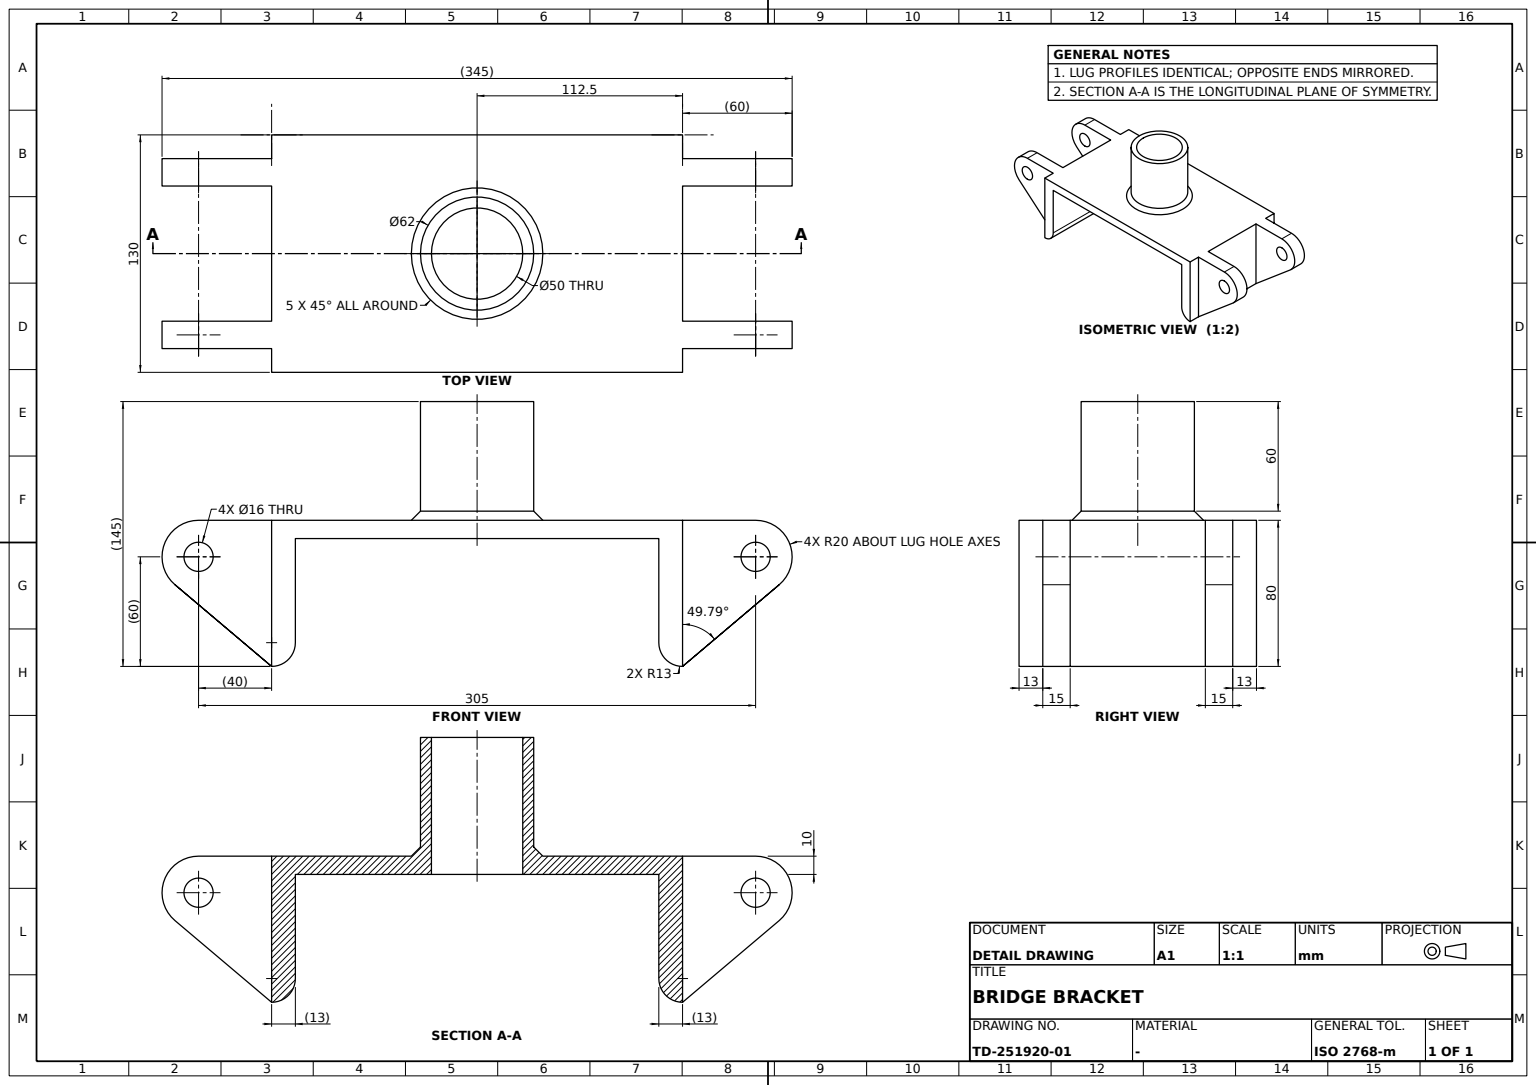
ISO-10303-21;
HEADER;
FILE_DESCRIPTION((''),'2;1');
FILE_NAME('','',(''),(''),'','','');
FILE_SCHEMA(('AUTOMOTIVE_DESIGN'));
ENDSEC;
DATA;
#1=APPLICATION_CONTEXT('');
#2=PRODUCT_CONTEXT('',#1,'mechanical');
#3=PRODUCT('','','',(#2));
#4=PRODUCT_DEFINITION_FORMATION('','',#3);
#5=PRODUCT_DEFINITION_CONTEXT('',#1,'design');
#6=PRODUCT_DEFINITION('','',#4,#5);
#7=PRODUCT_DEFINITION_SHAPE('','',#6);
#8=(LENGTH_UNIT()NAMED_UNIT(*)SI_UNIT(.MILLI.,.METRE.));
#9=(NAMED_UNIT(*)PLANE_ANGLE_UNIT()SI_UNIT($,.RADIAN.));
#10=(NAMED_UNIT(*)SI_UNIT($,.STERADIAN.)SOLID_ANGLE_UNIT());
#11=UNCERTAINTY_MEASURE_WITH_UNIT(LENGTH_MEASURE(0.005),#8,'distance_accuracy_value','');
#12=(GEOMETRIC_REPRESENTATION_CONTEXT(3)GLOBAL_UNCERTAINTY_ASSIGNED_CONTEXT((#11))GLOBAL_UNIT_ASSIGNED_CONTEXT((#8,#9,#10))REPRESENTATION_CONTEXT('',''));
#13=CARTESIAN_POINT('',(-25.,0.,-10.));
#14=VERTEX_POINT('',#13);
#15=CARTESIAN_POINT('',(25.,0.,-10.));
#16=VERTEX_POINT('',#15);
#17=CARTESIAN_POINT('',(0.,0.,-10.));
#18=DIRECTION('',(0.,0.,1.));
#19=DIRECTION('',(1.,0.,0.));
#20=AXIS2_PLACEMENT_3D('',#17,#18,#19);
#21=CIRCLE('',#20,25.);
#22=EDGE_CURVE('',#14,#16,#21,.T.);
#23=ORIENTED_EDGE('',*,*,#22,.F.);
#24=CARTESIAN_POINT('',(-25.,0.,65.));
#25=VERTEX_POINT('',#24);
#26=CARTESIAN_POINT('',(-25.,0.,0.));
#27=VECTOR('',#18,1000.);
#28=LINE('',#26,#27);
#29=EDGE_CURVE('',#14,#25,#28,.T.);
#30=ORIENTED_EDGE('',*,*,#29,.T.);
#31=CARTESIAN_POINT('',(25.,0.,65.));
#32=VERTEX_POINT('',#31);
#33=CARTESIAN_POINT('',(0.,0.,65.));
#34=AXIS2_PLACEMENT_3D('',#33,#18,#19);
#35=CIRCLE('',#34,25.);
#36=EDGE_CURVE('',#25,#32,#35,.T.);
#37=ORIENTED_EDGE('',*,*,#36,.T.);
#38=CARTESIAN_POINT('',(25.,0.,0.));
#39=LINE('',#38,#27);
#40=EDGE_CURVE('',#32,#16,#39,.F.);
#41=ORIENTED_EDGE('',*,*,#40,.T.);
#42=EDGE_LOOP('',(#23,#30,#37,#41));
#43=FACE_BOUND('',#42,.T.);
#44=CARTESIAN_POINT('',(0.,0.,0.));
#45=AXIS2_PLACEMENT_3D('',#44,#18,#19);
#46=CYLINDRICAL_SURFACE('',#45,25.);
#47=ADVANCED_FACE('',(#43),#46,.F.);
#48=CARTESIAN_POINT('',(165.411238,-37.,-35.274159));
#49=VERTEX_POINT('',#48);
#50=CARTESIAN_POINT('',(165.411238,-52.,-35.274159));
#51=VERTEX_POINT('',#50);
#52=DIRECTION('',(0.,-1.,0.));
#53=VECTOR('',#52,1000.);
#54=LINE('',#48,#53);
#55=EDGE_CURVE('',#49,#51,#54,.T.);
#56=ORIENTED_EDGE('',*,*,#55,.F.);
#57=CARTESIAN_POINT('',(152.5,-37.,0.));
#58=VERTEX_POINT('',#57);
#59=CARTESIAN_POINT('',(152.5,-37.,-20.));
#60=AXIS2_PLACEMENT_3D('',#59,#52,#19);
#61=CIRCLE('',#60,20.);
#62=EDGE_CURVE('',#49,#58,#61,.T.);
#63=ORIENTED_EDGE('',*,*,#62,.T.);
#64=CARTESIAN_POINT('',(152.5,-52.,0.));
#65=VERTEX_POINT('',#64);
#66=LINE('',#57,#53);
#67=EDGE_CURVE('',#58,#65,#66,.T.);
#68=ORIENTED_EDGE('',*,*,#67,.T.);
#69=CARTESIAN_POINT('',(152.5,-52.,-20.));
#70=AXIS2_PLACEMENT_3D('',#69,#52,#19);
#71=CIRCLE('',#70,20.);
#72=EDGE_CURVE('',#51,#65,#71,.T.);
#73=ORIENTED_EDGE('',*,*,#72,.F.);
#74=EDGE_LOOP('',(#56,#63,#68,#73));
#75=FACE_BOUND('',#74,.T.);
#76=DIRECTION('',(0.,0.,-1.));
#77=AXIS2_PLACEMENT_3D('',#59,#52,#76);
#78=CYLINDRICAL_SURFACE('',#77,20.);
#79=ADVANCED_FACE('',(#75),#78,.T.);
#80=CARTESIAN_POINT('',(152.5,37.,-12.));
#81=VERTEX_POINT('',#80);
#82=CARTESIAN_POINT('',(152.5,37.,-28.));
#83=VERTEX_POINT('',#82);
#84=CARTESIAN_POINT('',(152.5,37.,-20.));
#85=AXIS2_PLACEMENT_3D('',#84,#52,#19);
#86=CIRCLE('',#85,8.);
#87=EDGE_CURVE('',#81,#83,#86,.T.);
#88=ORIENTED_EDGE('',*,*,#87,.T.);
#89=CARTESIAN_POINT('',(152.5,52.,-28.));
#90=VERTEX_POINT('',#89);
#91=DIRECTION('',(0.,1.,0.));
#92=VECTOR('',#91,1000.);
#93=LINE('',#82,#92);
#94=EDGE_CURVE('',#83,#90,#93,.T.);
#95=ORIENTED_EDGE('',*,*,#94,.T.);
#96=CARTESIAN_POINT('',(152.5,52.,-12.));
#97=VERTEX_POINT('',#96);
#98=CARTESIAN_POINT('',(152.5,52.,-20.));
#99=AXIS2_PLACEMENT_3D('',#98,#52,#19);
#100=CIRCLE('',#99,8.);
#101=EDGE_CURVE('',#97,#90,#100,.T.);
#102=ORIENTED_EDGE('',*,*,#101,.F.);
#103=LINE('',#80,#92);
#104=EDGE_CURVE('',#97,#81,#103,.F.);
#105=ORIENTED_EDGE('',*,*,#104,.T.);
#106=EDGE_LOOP('',(#88,#95,#102,#105));
#107=FACE_BOUND('',#106,.T.);
#108=AXIS2_PLACEMENT_3D('',#84,#91,#18);
#109=CYLINDRICAL_SURFACE('',#108,8.);
#110=ADVANCED_FACE('',(#107),#109,.F.);
#111=EDGE_CURVE('',#32,#25,#35,.T.);
#112=ORIENTED_EDGE('',*,*,#111,.F.);
#113=ORIENTED_EDGE('',*,*,#36,.F.);
#114=EDGE_LOOP('',(#112,#113));
#115=FACE_BOUND('',#114,.T.);
#116=CARTESIAN_POINT('',(-31.,0.,65.));
#117=VERTEX_POINT('',#116);
#118=CARTESIAN_POINT('',(31.,0.,65.));
#119=VERTEX_POINT('',#118);
#120=CIRCLE('',#34,31.);
#121=EDGE_CURVE('',#117,#119,#120,.T.);
#122=ORIENTED_EDGE('',*,*,#121,.T.);
#123=EDGE_CURVE('',#119,#117,#120,.T.);
#124=ORIENTED_EDGE('',*,*,#123,.T.);
#125=EDGE_LOOP('',(#122,#124));
#126=FACE_BOUND('',#125,.T.);
#127=PLANE('',#34);
#128=ADVANCED_FACE('',(#115,#126),#127,.T.);
#129=CARTESIAN_POINT('',(-152.5,-37.,-28.));
#130=VERTEX_POINT('',#129);
#131=CARTESIAN_POINT('',(-152.5,-52.,-28.));
#132=VERTEX_POINT('',#131);
#133=LINE('',#129,#53);
#134=EDGE_CURVE('',#130,#132,#133,.T.);
#135=ORIENTED_EDGE('',*,*,#134,.T.);
#136=CARTESIAN_POINT('',(-152.5,-52.,-12.));
#137=VERTEX_POINT('',#136);
#138=CARTESIAN_POINT('',(-152.5,-52.,-20.));
#139=DIRECTION('',(-1.,0.,0.));
#140=AXIS2_PLACEMENT_3D('',#138,#91,#139);
#141=CIRCLE('',#140,8.);
#142=EDGE_CURVE('',#137,#132,#141,.T.);
#143=ORIENTED_EDGE('',*,*,#142,.F.);
#144=CARTESIAN_POINT('',(-152.5,-37.,-12.));
#145=VERTEX_POINT('',#144);
#146=LINE('',#144,#53);
#147=EDGE_CURVE('',#137,#145,#146,.F.);
#148=ORIENTED_EDGE('',*,*,#147,.T.);
#149=CARTESIAN_POINT('',(-152.5,-37.,-20.));
#150=AXIS2_PLACEMENT_3D('',#149,#91,#139);
#151=CIRCLE('',#150,8.);
#152=EDGE_CURVE('',#145,#130,#151,.T.);
#153=ORIENTED_EDGE('',*,*,#152,.T.);
#154=EDGE_LOOP('',(#135,#143,#148,#153));
#155=FACE_BOUND('',#154,.T.);
#156=AXIS2_PLACEMENT_3D('',#149,#52,#76);
#157=CYLINDRICAL_SURFACE('',#156,8.);
#158=ADVANCED_FACE('',(#155),#157,.F.);
#159=CARTESIAN_POINT('',(-152.5,37.,-12.));
#160=VERTEX_POINT('',#159);
#161=CARTESIAN_POINT('',(-152.5,37.,-28.));
#162=VERTEX_POINT('',#161);
#163=CARTESIAN_POINT('',(-152.5,37.,-20.));
#164=AXIS2_PLACEMENT_3D('',#163,#91,#139);
#165=CIRCLE('',#164,8.);
#166=EDGE_CURVE('',#160,#162,#165,.T.);
#167=ORIENTED_EDGE('',*,*,#166,.F.);
#168=CARTESIAN_POINT('',(-152.5,52.,-12.));
#169=VERTEX_POINT('',#168);
#170=LINE('',#159,#92);
#171=EDGE_CURVE('',#160,#169,#170,.T.);
#172=ORIENTED_EDGE('',*,*,#171,.T.);
#173=CARTESIAN_POINT('',(-152.5,52.,-28.));
#174=VERTEX_POINT('',#173);
#175=CARTESIAN_POINT('',(-152.5,52.,-20.));
#176=AXIS2_PLACEMENT_3D('',#175,#91,#139);
#177=CIRCLE('',#176,8.);
#178=EDGE_CURVE('',#169,#174,#177,.T.);
#179=ORIENTED_EDGE('',*,*,#178,.T.);
#180=LINE('',#161,#92);
#181=EDGE_CURVE('',#174,#162,#180,.F.);
#182=ORIENTED_EDGE('',*,*,#181,.T.);
#183=EDGE_LOOP('',(#167,#172,#179,#182));
#184=FACE_BOUND('',#183,.T.);
#185=AXIS2_PLACEMENT_3D('',#163,#91,#18);
#186=CYLINDRICAL_SURFACE('',#185,8.);
#187=ADVANCED_FACE('',(#184),#186,.F.);
#188=CARTESIAN_POINT('',(112.5,65.,-80.));
#189=VERTEX_POINT('',#188);
#190=CARTESIAN_POINT('',(112.5,65.,0.));
#191=VERTEX_POINT('',#190);
#192=LINE('',#188,#27);
#193=EDGE_CURVE('',#189,#191,#192,.T.);
#194=ORIENTED_EDGE('',*,*,#193,.F.);
#195=CARTESIAN_POINT('',(99.5,65.,-67.));
#196=VERTEX_POINT('',#195);
#197=CARTESIAN_POINT('',(112.5,65.,-67.));
#198=AXIS2_PLACEMENT_3D('',#197,#52,#19);
#199=CIRCLE('',#198,13.);
#200=EDGE_CURVE('',#196,#189,#199,.T.);
#201=ORIENTED_EDGE('',*,*,#200,.F.);
#202=CARTESIAN_POINT('',(99.5,65.,-10.));
#203=VERTEX_POINT('',#202);
#204=VECTOR('',#76,1000.);
#205=LINE('',#202,#204);
#206=EDGE_CURVE('',#203,#196,#205,.T.);
#207=ORIENTED_EDGE('',*,*,#206,.F.);
#208=CARTESIAN_POINT('',(-99.5,65.,-10.));
#209=VERTEX_POINT('',#208);
#210=VECTOR('',#19,1000.);
#211=LINE('',#208,#210);
#212=EDGE_CURVE('',#209,#203,#211,.T.);
#213=ORIENTED_EDGE('',*,*,#212,.F.);
#214=CARTESIAN_POINT('',(-99.5,65.,-67.));
#215=VERTEX_POINT('',#214);
#216=LINE('',#214,#27);
#217=EDGE_CURVE('',#215,#209,#216,.T.);
#218=ORIENTED_EDGE('',*,*,#217,.F.);
#219=CARTESIAN_POINT('',(-112.5,65.,-80.));
#220=VERTEX_POINT('',#219);
#221=CARTESIAN_POINT('',(-112.5,65.,-67.));
#222=AXIS2_PLACEMENT_3D('',#221,#52,#19);
#223=CIRCLE('',#222,13.);
#224=EDGE_CURVE('',#220,#215,#223,.T.);
#225=ORIENTED_EDGE('',*,*,#224,.F.);
#226=CARTESIAN_POINT('',(-112.5,65.,0.));
#227=VERTEX_POINT('',#226);
#228=LINE('',#226,#204);
#229=EDGE_CURVE('',#227,#220,#228,.T.);
#230=ORIENTED_EDGE('',*,*,#229,.F.);
#231=VECTOR('',#139,1000.);
#232=LINE('',#190,#231);
#233=EDGE_CURVE('',#191,#227,#232,.T.);
#234=ORIENTED_EDGE('',*,*,#233,.F.);
#235=EDGE_LOOP('',(#194,#201,#207,#213,#218,#225,#230,#234));
#236=FACE_BOUND('',#235,.T.);
#237=AXIS2_PLACEMENT_3D('',#221,#52,#76);
#238=PLANE('',#237);
#239=ADVANCED_FACE('',(#236),#238,.F.);
#240=ORIENTED_EDGE('',*,*,#181,.F.);
#241=EDGE_CURVE('',#174,#169,#177,.T.);
#242=ORIENTED_EDGE('',*,*,#241,.T.);
#243=ORIENTED_EDGE('',*,*,#171,.F.);
#244=EDGE_CURVE('',#162,#160,#165,.T.);
#245=ORIENTED_EDGE('',*,*,#244,.F.);
#246=EDGE_LOOP('',(#240,#242,#243,#245));
#247=FACE_BOUND('',#246,.T.);
#248=ADVANCED_FACE('',(#247),#186,.F.);
#249=CARTESIAN_POINT('',(112.5,-52.,-80.));
#250=VERTEX_POINT('',#249);
#251=DIRECTION('',(0.763707941,0.,0.645561911));
#252=VECTOR('',#251,1000.);
#253=LINE('',#249,#252);
#254=EDGE_CURVE('',#250,#51,#253,.T.);
#255=ORIENTED_EDGE('',*,*,#254,.F.);
#256=CARTESIAN_POINT('',(112.5,-37.,-80.));
#257=VERTEX_POINT('',#256);
#258=LINE('',#256,#53);
#259=EDGE_CURVE('',#257,#250,#258,.T.);
#260=ORIENTED_EDGE('',*,*,#259,.F.);
#261=LINE('',#256,#252);
#262=EDGE_CURVE('',#257,#49,#261,.T.);
#263=ORIENTED_EDGE('',*,*,#262,.T.);
#264=ORIENTED_EDGE('',*,*,#55,.T.);
#265=EDGE_LOOP('',(#255,#260,#263,#264));
#266=FACE_BOUND('',#265,.T.);
#267=DIRECTION('',(0.645561911,0.,-0.763707941));
#268=DIRECTION('',(-0.763707941,0.,-0.645561911));
#269=AXIS2_PLACEMENT_3D('',#256,#267,#268);
#270=PLANE('',#269);
#271=ADVANCED_FACE('',(#266),#270,.T.);
#272=CARTESIAN_POINT('',(152.5,-52.,-12.));
#273=VERTEX_POINT('',#272);
#274=CARTESIAN_POINT('',(152.5,-37.,-12.));
#275=VERTEX_POINT('',#274);
#276=LINE('',#274,#53);
#277=EDGE_CURVE('',#273,#275,#276,.F.);
#278=ORIENTED_EDGE('',*,*,#277,.F.);
#279=CARTESIAN_POINT('',(152.5,-52.,-28.));
#280=VERTEX_POINT('',#279);
#281=CIRCLE('',#70,8.);
#282=EDGE_CURVE('',#273,#280,#281,.T.);
#283=ORIENTED_EDGE('',*,*,#282,.T.);
#284=CARTESIAN_POINT('',(152.5,-37.,-28.));
#285=VERTEX_POINT('',#284);
#286=LINE('',#284,#53);
#287=EDGE_CURVE('',#285,#280,#286,.T.);
#288=ORIENTED_EDGE('',*,*,#287,.F.);
#289=CIRCLE('',#60,8.);
#290=EDGE_CURVE('',#275,#285,#289,.T.);
#291=ORIENTED_EDGE('',*,*,#290,.F.);
#292=EDGE_LOOP('',(#278,#283,#288,#291));
#293=FACE_BOUND('',#292,.T.);
#294=CYLINDRICAL_SURFACE('',#77,8.);
#295=ADVANCED_FACE('',(#293),#294,.F.);
#296=ORIENTED_EDGE('',*,*,#287,.T.);
#297=EDGE_CURVE('',#280,#273,#281,.T.);
#298=ORIENTED_EDGE('',*,*,#297,.T.);
#299=ORIENTED_EDGE('',*,*,#277,.T.);
#300=EDGE_CURVE('',#285,#275,#289,.T.);
#301=ORIENTED_EDGE('',*,*,#300,.F.);
#302=EDGE_LOOP('',(#296,#298,#299,#301));
#303=FACE_BOUND('',#302,.T.);
#304=ADVANCED_FACE('',(#303),#294,.F.);
#305=CARTESIAN_POINT('',(152.5,37.,0.));
#306=VERTEX_POINT('',#305);
#307=CARTESIAN_POINT('',(112.5,37.,0.));
#308=VERTEX_POINT('',#307);
#309=LINE('',#305,#231);
#310=EDGE_CURVE('',#306,#308,#309,.T.);
#311=ORIENTED_EDGE('',*,*,#310,.F.);
#312=CARTESIAN_POINT('',(152.5,52.,0.));
#313=VERTEX_POINT('',#312);
#314=LINE('',#305,#92);
#315=EDGE_CURVE('',#306,#313,#314,.T.);
#316=ORIENTED_EDGE('',*,*,#315,.T.);
#317=CARTESIAN_POINT('',(112.5,52.,0.));
#318=VERTEX_POINT('',#317);
#319=LINE('',#312,#231);
#320=EDGE_CURVE('',#313,#318,#319,.T.);
#321=ORIENTED_EDGE('',*,*,#320,.T.);
#322=CARTESIAN_POINT('',(112.5,-65.,0.));
#323=LINE('',#322,#92);
#324=EDGE_CURVE('',#318,#191,#323,.T.);
#325=ORIENTED_EDGE('',*,*,#324,.T.);
#326=ORIENTED_EDGE('',*,*,#233,.T.);
#327=CARTESIAN_POINT('',(-112.5,52.,0.));
#328=VERTEX_POINT('',#327);
#329=CARTESIAN_POINT('',(-112.5,-65.,0.));
#330=LINE('',#329,#92);
#331=EDGE_CURVE('',#328,#227,#330,.T.);
#332=ORIENTED_EDGE('',*,*,#331,.F.);
#333=CARTESIAN_POINT('',(-152.5,52.,0.));
#334=VERTEX_POINT('',#333);
#335=LINE('',#333,#210);
#336=EDGE_CURVE('',#334,#328,#335,.T.);
#337=ORIENTED_EDGE('',*,*,#336,.F.);
#338=CARTESIAN_POINT('',(-152.5,37.,0.));
#339=VERTEX_POINT('',#338);
#340=LINE('',#338,#92);
#341=EDGE_CURVE('',#339,#334,#340,.T.);
#342=ORIENTED_EDGE('',*,*,#341,.F.);
#343=CARTESIAN_POINT('',(-112.5,37.,0.));
#344=VERTEX_POINT('',#343);
#345=LINE('',#338,#210);
#346=EDGE_CURVE('',#339,#344,#345,.T.);
#347=ORIENTED_EDGE('',*,*,#346,.T.);
#348=CARTESIAN_POINT('',(-112.5,-37.,0.));
#349=VERTEX_POINT('',#348);
#350=EDGE_CURVE('',#349,#344,#330,.T.);
#351=ORIENTED_EDGE('',*,*,#350,.F.);
#352=CARTESIAN_POINT('',(-152.5,-37.,0.));
#353=VERTEX_POINT('',#352);
#354=LINE('',#352,#210);
#355=EDGE_CURVE('',#353,#349,#354,.T.);
#356=ORIENTED_EDGE('',*,*,#355,.F.);
#357=CARTESIAN_POINT('',(-152.5,-52.,0.));
#358=VERTEX_POINT('',#357);
#359=LINE('',#352,#53);
#360=EDGE_CURVE('',#353,#358,#359,.T.);
#361=ORIENTED_EDGE('',*,*,#360,.T.);
#362=CARTESIAN_POINT('',(-112.5,-52.,0.));
#363=VERTEX_POINT('',#362);
#364=LINE('',#357,#210);
#365=EDGE_CURVE('',#358,#363,#364,.T.);
#366=ORIENTED_EDGE('',*,*,#365,.T.);
#367=VERTEX_POINT('',#329);
#368=EDGE_CURVE('',#367,#363,#330,.T.);
#369=ORIENTED_EDGE('',*,*,#368,.F.);
#370=VERTEX_POINT('',#322);
#371=LINE('',#322,#231);
#372=EDGE_CURVE('',#370,#367,#371,.T.);
#373=ORIENTED_EDGE('',*,*,#372,.F.);
#374=CARTESIAN_POINT('',(112.5,-52.,0.));
#375=VERTEX_POINT('',#374);
#376=EDGE_CURVE('',#370,#375,#323,.T.);
#377=ORIENTED_EDGE('',*,*,#376,.T.);
#378=LINE('',#64,#231);
#379=EDGE_CURVE('',#65,#375,#378,.T.);
#380=ORIENTED_EDGE('',*,*,#379,.F.);
#381=ORIENTED_EDGE('',*,*,#67,.F.);
#382=CARTESIAN_POINT('',(112.5,-37.,0.));
#383=VERTEX_POINT('',#382);
#384=LINE('',#57,#231);
#385=EDGE_CURVE('',#58,#383,#384,.T.);
#386=ORIENTED_EDGE('',*,*,#385,.T.);
#387=EDGE_CURVE('',#383,#308,#323,.T.);
#388=ORIENTED_EDGE('',*,*,#387,.T.);
#389=EDGE_LOOP('',(#311,#316,#321,#325,#326,#332,#337,#342,#347,#351,#356,#361,#366,#369,#373,#377,#380,#381,#386,#388));
#390=FACE_BOUND('',#389,.T.);
#391=CARTESIAN_POINT('',(36.,0.,0.));
#392=VERTEX_POINT('',#391);
#393=CARTESIAN_POINT('',(-36.,0.,0.));
#394=VERTEX_POINT('',#393);
#395=AXIS2_PLACEMENT_3D('',#44,#76,#139);
#396=CIRCLE('',#395,36.);
#397=EDGE_CURVE('',#392,#394,#396,.T.);
#398=ORIENTED_EDGE('',*,*,#397,.T.);
#399=EDGE_CURVE('',#394,#392,#396,.T.);
#400=ORIENTED_EDGE('',*,*,#399,.T.);
#401=EDGE_LOOP('',(#398,#400));
#402=FACE_BOUND('',#401,.T.);
#403=AXIS2_PLACEMENT_3D('',#322,#76,#139);
#404=PLANE('',#403);
#405=ADVANCED_FACE('',(#390,#402),#404,.F.);
#406=ORIENTED_EDGE('',*,*,#399,.F.);
#407=CARTESIAN_POINT('',(-31.,0.,5.));
#408=VERTEX_POINT('',#407);
#409=DIRECTION('',(-0.707106781,0.,-0.707106781));
#410=VECTOR('',#409,1000.);
#411=LINE('',#407,#410);
#412=EDGE_CURVE('',#408,#394,#411,.T.);
#413=ORIENTED_EDGE('',*,*,#412,.F.);
#414=CARTESIAN_POINT('',(31.,0.,5.));
#415=VERTEX_POINT('',#414);
#416=CARTESIAN_POINT('',(0.,0.,5.));
#417=AXIS2_PLACEMENT_3D('',#416,#18,#139);
#418=CIRCLE('',#417,31.);
#419=EDGE_CURVE('',#415,#408,#418,.T.);
#420=ORIENTED_EDGE('',*,*,#419,.F.);
#421=DIRECTION('',(0.707106781,0.,-0.707106781));
#422=VECTOR('',#421,1000.);
#423=LINE('',#414,#422);
#424=EDGE_CURVE('',#392,#415,#423,.F.);
#425=ORIENTED_EDGE('',*,*,#424,.F.);
#426=EDGE_LOOP('',(#406,#413,#420,#425));
#427=FACE_BOUND('',#426,.T.);
#428=AXIS2_PLACEMENT_3D('',#416,#76,#139);
#429=CONICAL_SURFACE('',#428,31.,0.785398163);
#430=ADVANCED_FACE('',(#427),#429,.T.);
#431=CARTESIAN_POINT('',(99.5,-65.,-10.));
#432=VERTEX_POINT('',#431);
#433=LINE('',#431,#92);
#434=EDGE_CURVE('',#432,#203,#433,.T.);
#435=ORIENTED_EDGE('',*,*,#434,.F.);
#436=CARTESIAN_POINT('',(-99.5,-65.,-10.));
#437=VERTEX_POINT('',#436);
#438=LINE('',#436,#210);
#439=EDGE_CURVE('',#437,#432,#438,.T.);
#440=ORIENTED_EDGE('',*,*,#439,.F.);
#441=LINE('',#436,#92);
#442=EDGE_CURVE('',#437,#209,#441,.T.);
#443=ORIENTED_EDGE('',*,*,#442,.T.);
#444=ORIENTED_EDGE('',*,*,#212,.T.);
#445=EDGE_LOOP('',(#435,#440,#443,#444));
#446=FACE_BOUND('',#445,.T.);
#447=EDGE_CURVE('',#16,#14,#21,.T.);
#448=ORIENTED_EDGE('',*,*,#447,.T.);
#449=ORIENTED_EDGE('',*,*,#22,.T.);
#450=EDGE_LOOP('',(#448,#449));
#451=FACE_BOUND('',#450,.T.);
#452=AXIS2_PLACEMENT_3D('',#436,#18,#19);
#453=PLANE('',#452);
#454=ADVANCED_FACE('',(#446,#451),#453,.F.);
#455=CARTESIAN_POINT('',(112.5,37.,-80.));
#456=VERTEX_POINT('',#455);
#457=CARTESIAN_POINT('',(112.5,-65.,-80.));
#458=LINE('',#457,#92);
#459=EDGE_CURVE('',#257,#456,#458,.T.);
#460=ORIENTED_EDGE('',*,*,#459,.T.);
#461=LINE('',#307,#204);
#462=EDGE_CURVE('',#308,#456,#461,.T.);
#463=ORIENTED_EDGE('',*,*,#462,.F.);
#464=ORIENTED_EDGE('',*,*,#387,.F.);
#465=LINE('',#382,#204);
#466=EDGE_CURVE('',#383,#257,#465,.T.);
#467=ORIENTED_EDGE('',*,*,#466,.T.);
#468=EDGE_LOOP('',(#460,#463,#464,#467));
#469=FACE_BOUND('',#468,.T.);
#470=AXIS2_PLACEMENT_3D('',#457,#139,#18);
#471=PLANE('',#470);
#472=ADVANCED_FACE('',(#469),#471,.F.);
#473=ORIENTED_EDGE('',*,*,#62,.F.);
#474=ORIENTED_EDGE('',*,*,#262,.F.);
#475=ORIENTED_EDGE('',*,*,#466,.F.);
#476=ORIENTED_EDGE('',*,*,#385,.F.);
#477=EDGE_LOOP('',(#473,#474,#475,#476));
#478=FACE_BOUND('',#477,.T.);
#479=ORIENTED_EDGE('',*,*,#290,.T.);
#480=ORIENTED_EDGE('',*,*,#300,.T.);
#481=EDGE_LOOP('',(#479,#480));
#482=FACE_BOUND('',#481,.T.);
#483=PLANE('',#77);
#484=ADVANCED_FACE('',(#478,#482),#483,.F.);
#485=CARTESIAN_POINT('',(165.411238,52.,-35.274159));
#486=VERTEX_POINT('',#485);
#487=CIRCLE('',#99,20.);
#488=EDGE_CURVE('',#486,#313,#487,.T.);
#489=ORIENTED_EDGE('',*,*,#488,.F.);
#490=CARTESIAN_POINT('',(112.5,52.,-80.));
#491=VERTEX_POINT('',#490);
#492=LINE('',#490,#252);
#493=EDGE_CURVE('',#491,#486,#492,.T.);
#494=ORIENTED_EDGE('',*,*,#493,.F.);
#495=LINE('',#317,#204);
#496=EDGE_CURVE('',#318,#491,#495,.T.);
#497=ORIENTED_EDGE('',*,*,#496,.F.);
#498=ORIENTED_EDGE('',*,*,#320,.F.);
#499=EDGE_LOOP('',(#489,#494,#497,#498));
#500=FACE_BOUND('',#499,.T.);
#501=EDGE_CURVE('',#90,#97,#100,.T.);
#502=ORIENTED_EDGE('',*,*,#501,.T.);
#503=ORIENTED_EDGE('',*,*,#101,.T.);
#504=EDGE_LOOP('',(#502,#503));
#505=FACE_BOUND('',#504,.T.);
#506=AXIS2_PLACEMENT_3D('',#98,#52,#76);
#507=PLANE('',#506);
#508=ADVANCED_FACE('',(#500,#505),#507,.F.);
#509=ORIENTED_EDGE('',*,*,#147,.F.);
#510=EDGE_CURVE('',#132,#137,#141,.T.);
#511=ORIENTED_EDGE('',*,*,#510,.F.);
#512=ORIENTED_EDGE('',*,*,#134,.F.);
#513=EDGE_CURVE('',#130,#145,#151,.T.);
#514=ORIENTED_EDGE('',*,*,#513,.T.);
#515=EDGE_LOOP('',(#509,#511,#512,#514));
#516=FACE_BOUND('',#515,.T.);
#517=ADVANCED_FACE('',(#516),#157,.F.);
#518=ORIENTED_EDGE('',*,*,#341,.T.);
#519=CARTESIAN_POINT('',(-165.411238,52.,-35.274159));
#520=VERTEX_POINT('',#519);
#521=CIRCLE('',#176,20.);
#522=EDGE_CURVE('',#520,#334,#521,.T.);
#523=ORIENTED_EDGE('',*,*,#522,.F.);
#524=CARTESIAN_POINT('',(-165.411238,37.,-35.274159));
#525=VERTEX_POINT('',#524);
#526=LINE('',#524,#92);
#527=EDGE_CURVE('',#525,#520,#526,.T.);
#528=ORIENTED_EDGE('',*,*,#527,.F.);
#529=CIRCLE('',#164,20.);
#530=EDGE_CURVE('',#525,#339,#529,.T.);
#531=ORIENTED_EDGE('',*,*,#530,.T.);
#532=EDGE_LOOP('',(#518,#523,#528,#531));
#533=FACE_BOUND('',#532,.T.);
#534=CYLINDRICAL_SURFACE('',#185,20.);
#535=ADVANCED_FACE('',(#533),#534,.T.);
#536=CARTESIAN_POINT('',(-112.5,-37.,-80.));
#537=VERTEX_POINT('',#536);
#538=LINE('',#348,#204);
#539=EDGE_CURVE('',#349,#537,#538,.T.);
#540=ORIENTED_EDGE('',*,*,#539,.F.);
#541=ORIENTED_EDGE('',*,*,#350,.T.);
#542=CARTESIAN_POINT('',(-112.5,37.,-80.));
#543=VERTEX_POINT('',#542);
#544=LINE('',#343,#204);
#545=EDGE_CURVE('',#344,#543,#544,.T.);
#546=ORIENTED_EDGE('',*,*,#545,.T.);
#547=CARTESIAN_POINT('',(-112.5,-65.,-80.));
#548=LINE('',#547,#92);
#549=EDGE_CURVE('',#537,#543,#548,.T.);
#550=ORIENTED_EDGE('',*,*,#549,.F.);
#551=EDGE_LOOP('',(#540,#541,#546,#550));
#552=FACE_BOUND('',#551,.T.);
#553=AXIS2_PLACEMENT_3D('',#329,#19,#76);
#554=PLANE('',#553);
#555=ADVANCED_FACE('',(#552),#554,.F.);
#556=ORIENTED_EDGE('',*,*,#200,.T.);
#557=EDGE_CURVE('',#491,#189,#458,.T.);
#558=ORIENTED_EDGE('',*,*,#557,.F.);
#559=LINE('',#455,#92);
#560=EDGE_CURVE('',#456,#491,#559,.T.);
#561=ORIENTED_EDGE('',*,*,#560,.F.);
#562=ORIENTED_EDGE('',*,*,#459,.F.);
#563=ORIENTED_EDGE('',*,*,#259,.T.);
#564=VERTEX_POINT('',#457);
#565=EDGE_CURVE('',#564,#250,#458,.T.);
#566=ORIENTED_EDGE('',*,*,#565,.F.);
#567=CARTESIAN_POINT('',(99.5,-65.,-67.));
#568=VERTEX_POINT('',#567);
#569=CARTESIAN_POINT('',(112.5,-65.,-67.));
#570=AXIS2_PLACEMENT_3D('',#569,#52,#19);
#571=CIRCLE('',#570,13.);
#572=EDGE_CURVE('',#568,#564,#571,.T.);
#573=ORIENTED_EDGE('',*,*,#572,.F.);
#574=LINE('',#567,#92);
#575=EDGE_CURVE('',#568,#196,#574,.T.);
#576=ORIENTED_EDGE('',*,*,#575,.T.);
#577=EDGE_LOOP('',(#556,#558,#561,#562,#563,#566,#573,#576));
#578=FACE_BOUND('',#577,.T.);
#579=AXIS2_PLACEMENT_3D('',#569,#91,#18);
#580=CYLINDRICAL_SURFACE('',#579,13.);
#581=ADVANCED_FACE('',(#578),#580,.T.);
#582=VERTEX_POINT('',#547);
#583=LINE('',#329,#204);
#584=EDGE_CURVE('',#367,#582,#583,.T.);
#585=ORIENTED_EDGE('',*,*,#584,.F.);
#586=ORIENTED_EDGE('',*,*,#368,.T.);
#587=CARTESIAN_POINT('',(-112.5,-52.,-80.));
#588=VERTEX_POINT('',#587);
#589=LINE('',#362,#204);
#590=EDGE_CURVE('',#363,#588,#589,.T.);
#591=ORIENTED_EDGE('',*,*,#590,.T.);
#592=EDGE_CURVE('',#582,#588,#548,.T.);
#593=ORIENTED_EDGE('',*,*,#592,.F.);
#594=EDGE_LOOP('',(#585,#586,#591,#593));
#595=FACE_BOUND('',#594,.T.);
#596=ADVANCED_FACE('',(#595),#554,.F.);
#597=LINE('',#374,#204);
#598=EDGE_CURVE('',#375,#250,#597,.T.);
#599=ORIENTED_EDGE('',*,*,#598,.F.);
#600=ORIENTED_EDGE('',*,*,#376,.F.);
#601=LINE('',#457,#27);
#602=EDGE_CURVE('',#564,#370,#601,.T.);
#603=ORIENTED_EDGE('',*,*,#602,.F.);
#604=ORIENTED_EDGE('',*,*,#565,.T.);
#605=EDGE_LOOP('',(#599,#600,#603,#604));
#606=FACE_BOUND('',#605,.T.);
#607=ADVANCED_FACE('',(#606),#471,.F.);
#608=ORIENTED_EDGE('',*,*,#87,.F.);
#609=EDGE_CURVE('',#83,#81,#86,.T.);
#610=ORIENTED_EDGE('',*,*,#609,.F.);
#611=EDGE_LOOP('',(#608,#610));
#612=FACE_BOUND('',#611,.T.);
#613=ORIENTED_EDGE('',*,*,#462,.T.);
#614=CARTESIAN_POINT('',(165.411238,37.,-35.274159));
#615=VERTEX_POINT('',#614);
#616=LINE('',#455,#252);
#617=EDGE_CURVE('',#456,#615,#616,.T.);
#618=ORIENTED_EDGE('',*,*,#617,.T.);
#619=CIRCLE('',#85,20.);
#620=EDGE_CURVE('',#615,#306,#619,.T.);
#621=ORIENTED_EDGE('',*,*,#620,.T.);
#622=ORIENTED_EDGE('',*,*,#310,.T.);
#623=EDGE_LOOP('',(#613,#618,#621,#622));
#624=FACE_BOUND('',#623,.T.);
#625=AXIS2_PLACEMENT_3D('',#84,#52,#76);
#626=PLANE('',#625);
#627=ADVANCED_FACE('',(#612,#624),#626,.T.);
#628=ORIENTED_EDGE('',*,*,#72,.T.);
#629=ORIENTED_EDGE('',*,*,#379,.T.);
#630=ORIENTED_EDGE('',*,*,#598,.T.);
#631=ORIENTED_EDGE('',*,*,#254,.T.);
#632=EDGE_LOOP('',(#628,#629,#630,#631));
#633=FACE_BOUND('',#632,.T.);
#634=ORIENTED_EDGE('',*,*,#297,.F.);
#635=ORIENTED_EDGE('',*,*,#282,.F.);
#636=EDGE_LOOP('',(#634,#635));
#637=FACE_BOUND('',#636,.T.);
#638=AXIS2_PLACEMENT_3D('',#69,#52,#76);
#639=PLANE('',#638);
#640=ADVANCED_FACE('',(#633,#637),#639,.T.);
#641=ORIENTED_EDGE('',*,*,#442,.F.);
#642=CARTESIAN_POINT('',(-99.5,-65.,-67.));
#643=VERTEX_POINT('',#642);
#644=LINE('',#642,#27);
#645=EDGE_CURVE('',#643,#437,#644,.T.);
#646=ORIENTED_EDGE('',*,*,#645,.F.);
#647=LINE('',#642,#92);
#648=EDGE_CURVE('',#643,#215,#647,.T.);
#649=ORIENTED_EDGE('',*,*,#648,.T.);
#650=ORIENTED_EDGE('',*,*,#217,.T.);
#651=EDGE_LOOP('',(#641,#646,#649,#650));
#652=FACE_BOUND('',#651,.T.);
#653=AXIS2_PLACEMENT_3D('',#642,#139,#18);
#654=PLANE('',#653);
#655=ADVANCED_FACE('',(#652),#654,.F.);
#656=ORIENTED_EDGE('',*,*,#360,.F.);
#657=CARTESIAN_POINT('',(-165.411238,-37.,-35.274159));
#658=VERTEX_POINT('',#657);
#659=CIRCLE('',#150,20.);
#660=EDGE_CURVE('',#658,#353,#659,.T.);
#661=ORIENTED_EDGE('',*,*,#660,.F.);
#662=CARTESIAN_POINT('',(-165.411238,-52.,-35.274159));
#663=VERTEX_POINT('',#662);
#664=LINE('',#657,#53);
#665=EDGE_CURVE('',#658,#663,#664,.T.);
#666=ORIENTED_EDGE('',*,*,#665,.T.);
#667=CIRCLE('',#140,20.);
#668=EDGE_CURVE('',#663,#358,#667,.T.);
#669=ORIENTED_EDGE('',*,*,#668,.T.);
#670=EDGE_LOOP('',(#656,#661,#666,#669));
#671=FACE_BOUND('',#670,.T.);
#672=CYLINDRICAL_SURFACE('',#156,20.);
#673=ADVANCED_FACE('',(#671),#672,.T.);
#674=ORIENTED_EDGE('',*,*,#244,.T.);
#675=ORIENTED_EDGE('',*,*,#166,.T.);
#676=EDGE_LOOP('',(#674,#675));
#677=FACE_BOUND('',#676,.T.);
#678=ORIENTED_EDGE('',*,*,#530,.F.);
#679=DIRECTION('',(-0.763707941,0.,0.645561911));
#680=VECTOR('',#679,1000.);
#681=LINE('',#542,#680);
#682=EDGE_CURVE('',#543,#525,#681,.T.);
#683=ORIENTED_EDGE('',*,*,#682,.F.);
#684=ORIENTED_EDGE('',*,*,#545,.F.);
#685=ORIENTED_EDGE('',*,*,#346,.F.);
#686=EDGE_LOOP('',(#678,#683,#684,#685));
#687=FACE_BOUND('',#686,.T.);
#688=PLANE('',#185);
#689=ADVANCED_FACE('',(#677,#687),#688,.F.);
#690=ORIENTED_EDGE('',*,*,#331,.T.);
#691=ORIENTED_EDGE('',*,*,#229,.T.);
#692=CARTESIAN_POINT('',(-112.5,52.,-80.));
#693=VERTEX_POINT('',#692);
#694=EDGE_CURVE('',#693,#220,#548,.T.);
#695=ORIENTED_EDGE('',*,*,#694,.F.);
#696=LINE('',#327,#204);
#697=EDGE_CURVE('',#328,#693,#696,.T.);
#698=ORIENTED_EDGE('',*,*,#697,.F.);
#699=EDGE_LOOP('',(#690,#691,#695,#698));
#700=FACE_BOUND('',#699,.T.);
#701=ADVANCED_FACE('',(#700),#554,.F.);
#702=ORIENTED_EDGE('',*,*,#111,.T.);
#703=ORIENTED_EDGE('',*,*,#29,.F.);
#704=ORIENTED_EDGE('',*,*,#447,.F.);
#705=ORIENTED_EDGE('',*,*,#40,.F.);
#706=EDGE_LOOP('',(#702,#703,#704,#705));
#707=FACE_BOUND('',#706,.T.);
#708=ADVANCED_FACE('',(#707),#46,.F.);
#709=ORIENTED_EDGE('',*,*,#697,.T.);
#710=LINE('',#692,#680);
#711=EDGE_CURVE('',#693,#520,#710,.T.);
#712=ORIENTED_EDGE('',*,*,#711,.T.);
#713=ORIENTED_EDGE('',*,*,#522,.T.);
#714=ORIENTED_EDGE('',*,*,#336,.T.);
#715=EDGE_LOOP('',(#709,#712,#713,#714));
#716=FACE_BOUND('',#715,.T.);
#717=ORIENTED_EDGE('',*,*,#178,.F.);
#718=ORIENTED_EDGE('',*,*,#241,.F.);
#719=EDGE_LOOP('',(#717,#718));
#720=FACE_BOUND('',#719,.T.);
#721=AXIS2_PLACEMENT_3D('',#175,#91,#18);
#722=PLANE('',#721);
#723=ADVANCED_FACE('',(#716,#720),#722,.T.);
#724=ORIENTED_EDGE('',*,*,#527,.T.);
#725=ORIENTED_EDGE('',*,*,#711,.F.);
#726=LINE('',#542,#92);
#727=EDGE_CURVE('',#543,#693,#726,.T.);
#728=ORIENTED_EDGE('',*,*,#727,.F.);
#729=ORIENTED_EDGE('',*,*,#682,.T.);
#730=EDGE_LOOP('',(#724,#725,#728,#729));
#731=FACE_BOUND('',#730,.T.);
#732=DIRECTION('',(-0.645561911,0.,-0.763707941));
#733=AXIS2_PLACEMENT_3D('',#542,#732,#679);
#734=PLANE('',#733);
#735=ADVANCED_FACE('',(#731),#734,.T.);
#736=ORIENTED_EDGE('',*,*,#668,.F.);
#737=LINE('',#587,#680);
#738=EDGE_CURVE('',#588,#663,#737,.T.);
#739=ORIENTED_EDGE('',*,*,#738,.F.);
#740=ORIENTED_EDGE('',*,*,#590,.F.);
#741=ORIENTED_EDGE('',*,*,#365,.F.);
#742=EDGE_LOOP('',(#736,#739,#740,#741));
#743=FACE_BOUND('',#742,.T.);
#744=ORIENTED_EDGE('',*,*,#142,.T.);
#745=ORIENTED_EDGE('',*,*,#510,.T.);
#746=EDGE_LOOP('',(#744,#745));
#747=FACE_BOUND('',#746,.T.);
#748=AXIS2_PLACEMENT_3D('',#138,#91,#18);
#749=PLANE('',#748);
#750=ADVANCED_FACE('',(#743,#747),#749,.F.);
#751=ORIENTED_EDGE('',*,*,#488,.T.);
#752=ORIENTED_EDGE('',*,*,#315,.F.);
#753=ORIENTED_EDGE('',*,*,#620,.F.);
#754=LINE('',#614,#92);
#755=EDGE_CURVE('',#615,#486,#754,.T.);
#756=ORIENTED_EDGE('',*,*,#755,.T.);
#757=EDGE_LOOP('',(#751,#752,#753,#756));
#758=FACE_BOUND('',#757,.T.);
#759=CYLINDRICAL_SURFACE('',#108,20.);
#760=ADVANCED_FACE('',(#758),#759,.T.);
#761=LINE('',#431,#204);
#762=EDGE_CURVE('',#432,#568,#761,.T.);
#763=ORIENTED_EDGE('',*,*,#762,.F.);
#764=ORIENTED_EDGE('',*,*,#434,.T.);
#765=ORIENTED_EDGE('',*,*,#206,.T.);
#766=ORIENTED_EDGE('',*,*,#575,.F.);
#767=EDGE_LOOP('',(#763,#764,#765,#766));
#768=FACE_BOUND('',#767,.T.);
#769=AXIS2_PLACEMENT_3D('',#431,#19,#76);
#770=PLANE('',#769);
#771=ADVANCED_FACE('',(#768),#770,.F.);
#772=ORIENTED_EDGE('',*,*,#592,.T.);
#773=LINE('',#536,#53);
#774=EDGE_CURVE('',#537,#588,#773,.T.);
#775=ORIENTED_EDGE('',*,*,#774,.F.);
#776=ORIENTED_EDGE('',*,*,#549,.T.);
#777=ORIENTED_EDGE('',*,*,#727,.T.);
#778=ORIENTED_EDGE('',*,*,#694,.T.);
#779=ORIENTED_EDGE('',*,*,#224,.T.);
#780=ORIENTED_EDGE('',*,*,#648,.F.);
#781=CARTESIAN_POINT('',(-112.5,-65.,-67.));
#782=AXIS2_PLACEMENT_3D('',#781,#52,#19);
#783=CIRCLE('',#782,13.);
#784=EDGE_CURVE('',#582,#643,#783,.T.);
#785=ORIENTED_EDGE('',*,*,#784,.F.);
#786=EDGE_LOOP('',(#772,#775,#776,#777,#778,#779,#780,#785));
#787=FACE_BOUND('',#786,.T.);
#788=AXIS2_PLACEMENT_3D('',#781,#91,#18);
#789=CYLINDRICAL_SURFACE('',#788,13.);
#790=ADVANCED_FACE('',(#787),#789,.T.);
#791=ORIENTED_EDGE('',*,*,#123,.F.);
#792=CARTESIAN_POINT('',(31.,0.,0.));
#793=LINE('',#792,#27);
#794=EDGE_CURVE('',#415,#119,#793,.T.);
#795=ORIENTED_EDGE('',*,*,#794,.F.);
#796=ORIENTED_EDGE('',*,*,#419,.T.);
#797=CARTESIAN_POINT('',(-31.,0.,0.));
#798=LINE('',#797,#27);
#799=EDGE_CURVE('',#117,#408,#798,.F.);
#800=ORIENTED_EDGE('',*,*,#799,.F.);
#801=EDGE_LOOP('',(#791,#795,#796,#800));
#802=FACE_BOUND('',#801,.T.);
#803=CYLINDRICAL_SURFACE('',#45,31.);
#804=ADVANCED_FACE('',(#802),#803,.T.);
#805=LINE('',#536,#680);
#806=EDGE_CURVE('',#537,#658,#805,.T.);
#807=ORIENTED_EDGE('',*,*,#806,.T.);
#808=ORIENTED_EDGE('',*,*,#660,.T.);
#809=ORIENTED_EDGE('',*,*,#355,.T.);
#810=ORIENTED_EDGE('',*,*,#539,.T.);
#811=EDGE_LOOP('',(#807,#808,#809,#810));
#812=FACE_BOUND('',#811,.T.);
#813=ORIENTED_EDGE('',*,*,#152,.F.);
#814=ORIENTED_EDGE('',*,*,#513,.F.);
#815=EDGE_LOOP('',(#813,#814));
#816=FACE_BOUND('',#815,.T.);
#817=AXIS2_PLACEMENT_3D('',#149,#91,#18);
#818=PLANE('',#817);
#819=ADVANCED_FACE('',(#812,#816),#818,.T.);
#820=ORIENTED_EDGE('',*,*,#121,.F.);
#821=ORIENTED_EDGE('',*,*,#799,.T.);
#822=EDGE_CURVE('',#408,#415,#418,.T.);
#823=ORIENTED_EDGE('',*,*,#822,.T.);
#824=ORIENTED_EDGE('',*,*,#794,.T.);
#825=EDGE_LOOP('',(#820,#821,#823,#824));
#826=FACE_BOUND('',#825,.T.);
#827=ADVANCED_FACE('',(#826),#803,.T.);
#828=ORIENTED_EDGE('',*,*,#609,.T.);
#829=ORIENTED_EDGE('',*,*,#104,.F.);
#830=ORIENTED_EDGE('',*,*,#501,.F.);
#831=ORIENTED_EDGE('',*,*,#94,.F.);
#832=EDGE_LOOP('',(#828,#829,#830,#831));
#833=FACE_BOUND('',#832,.T.);
#834=ADVANCED_FACE('',(#833),#109,.F.);
#835=ORIENTED_EDGE('',*,*,#193,.T.);
#836=ORIENTED_EDGE('',*,*,#324,.F.);
#837=ORIENTED_EDGE('',*,*,#496,.T.);
#838=ORIENTED_EDGE('',*,*,#557,.T.);
#839=EDGE_LOOP('',(#835,#836,#837,#838));
#840=FACE_BOUND('',#839,.T.);
#841=ADVANCED_FACE('',(#840),#471,.F.);
#842=ORIENTED_EDGE('',*,*,#822,.F.);
#843=ORIENTED_EDGE('',*,*,#412,.T.);
#844=ORIENTED_EDGE('',*,*,#397,.F.);
#845=ORIENTED_EDGE('',*,*,#424,.T.);
#846=EDGE_LOOP('',(#842,#843,#844,#845));
#847=FACE_BOUND('',#846,.T.);
#848=ADVANCED_FACE('',(#847),#429,.T.);
#849=ORIENTED_EDGE('',*,*,#755,.F.);
#850=ORIENTED_EDGE('',*,*,#617,.F.);
#851=ORIENTED_EDGE('',*,*,#560,.T.);
#852=ORIENTED_EDGE('',*,*,#493,.T.);
#853=EDGE_LOOP('',(#849,#850,#851,#852));
#854=FACE_BOUND('',#853,.T.);
#855=DIRECTION('',(-0.645561911,0.,0.763707941));
#856=AXIS2_PLACEMENT_3D('',#455,#855,#251);
#857=PLANE('',#856);
#858=ADVANCED_FACE('',(#854),#857,.F.);
#859=ORIENTED_EDGE('',*,*,#645,.T.);
#860=ORIENTED_EDGE('',*,*,#439,.T.);
#861=ORIENTED_EDGE('',*,*,#762,.T.);
#862=ORIENTED_EDGE('',*,*,#572,.T.);
#863=ORIENTED_EDGE('',*,*,#602,.T.);
#864=ORIENTED_EDGE('',*,*,#372,.T.);
#865=ORIENTED_EDGE('',*,*,#584,.T.);
#866=ORIENTED_EDGE('',*,*,#784,.T.);
#867=EDGE_LOOP('',(#859,#860,#861,#862,#863,#864,#865,#866));
#868=FACE_BOUND('',#867,.T.);
#869=AXIS2_PLACEMENT_3D('',#781,#52,#76);
#870=PLANE('',#869);
#871=ADVANCED_FACE('',(#868),#870,.T.);
#872=ORIENTED_EDGE('',*,*,#738,.T.);
#873=ORIENTED_EDGE('',*,*,#665,.F.);
#874=ORIENTED_EDGE('',*,*,#806,.F.);
#875=ORIENTED_EDGE('',*,*,#774,.T.);
#876=EDGE_LOOP('',(#872,#873,#874,#875));
#877=FACE_BOUND('',#876,.T.);
#878=DIRECTION('',(0.645561911,0.,0.763707941));
#879=DIRECTION('',(0.763707941,0.,-0.645561911));
#880=AXIS2_PLACEMENT_3D('',#536,#878,#879);
#881=PLANE('',#880);
#882=ADVANCED_FACE('',(#877),#881,.F.);
#883=CLOSED_SHELL('',(#47,#79,#110,#128,#158,#187,#239,#248,#271,#295,#304,#405,#430,#454,#472,#484,#508,#517,#535,#555,#581,#596,#607,#627,#640,#655,#673,#689,#701,#708,#723,#735,#750,#760,#771,#790,#804,#819,#827,#834,#841,#848,#858,#871,#882));
#884=MANIFOLD_SOLID_BREP('',#883);
#885=ADVANCED_BREP_SHAPE_REPRESENTATION('',(#884),#12);
#886=SHAPE_DEFINITION_REPRESENTATION(#7,#885);
ENDSEC;
END-ISO-10303-21;
